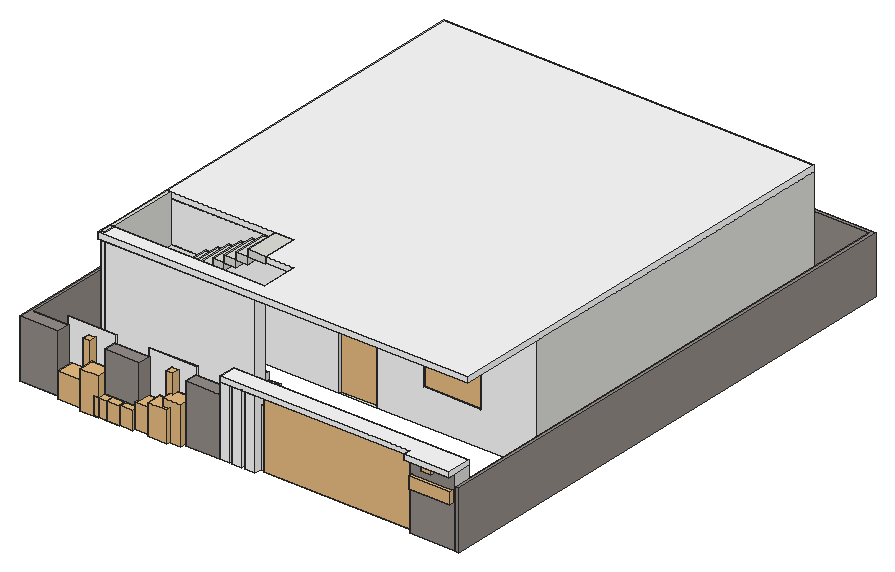
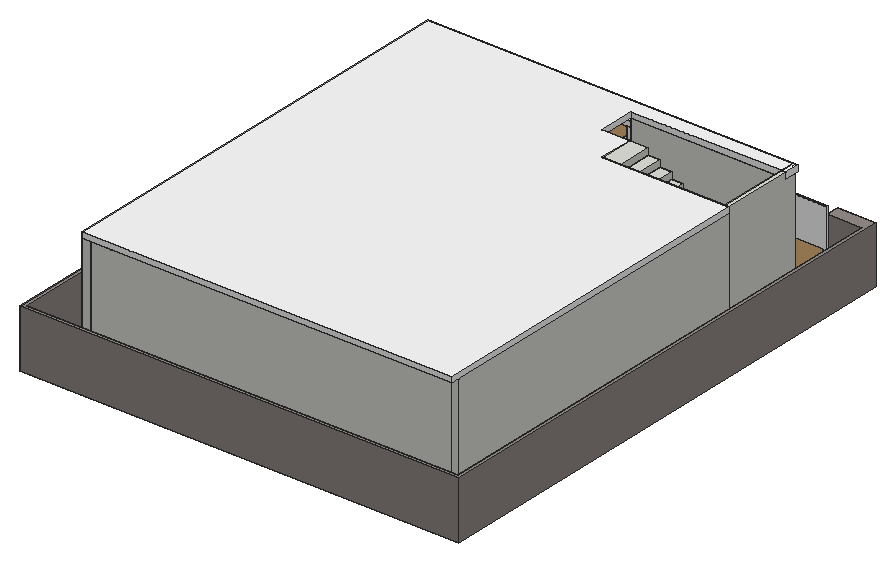
# SketchUp Ruby script. Lengths in inches.
U = 1.inch
M = Sketchup.active_model
def pt(a) = Geom::Point3d.new(a.map { |v| v * U })
def face(e, loops, mat)
  f = e.add_face(loops[0].map { |a| pt(a) })
  loops[1..].each { |l| e.add_face(l.map { |a| pt(a) }).erase! }
  f.material = f.back_material = mat if mat
  f
end
# faces: each face lists its corners as indices into pts; further lists are holes
def faces(e, pts, list, mat = nil) = list.each { |f| face(e, (f[0].is_a?(Array) ? f : [f]).map { |l| l.map { |i| pts[i] } }, mat) }
# xy, xz, yz: faces in a plane at the given z, y or x. An outline is a flat list of corners, or four numbers for a rectangle; further outlines are holes
def ring(l) = l.size == 4 ? [[l[0], l[1]], [l[2], l[1]], [l[2], l[3]], [l[0], l[3]]] : l.each_slice(2).to_a
def flat(e, list, mat, &to3) = list.each { |f| face(e, (f[0].is_a?(Array) ? f : [f]).map { |l| ring(l).map { |u, v| to3.(u, v) } }, mat) }
def xy(e, z, list, mat = nil) = flat(e, list, mat) { |x, y| [x, y, z] }
def xz(e, y, list, mat = nil) = flat(e, list, mat) { |x, z| [x, y, z] }
def yz(e, x, list, mat = nil) = flat(e, list, mat) { |y, z| [x, y, z] }
def lines(e, pts, list) = list.each { |a, b| e.add_line(pt(pts[a]), pt(pts[b])) }
# prism: a flat outline (further loops are holes) pulled along v
def prism(e, loops, v, mat = nil)
  f = face(e, loops, mat); d = Geom::Vector3d.new(v.map { |x| x * U })
  f.pushpull(f.normal.samedirection?(d) ? d.length : -d.length)
end
def box(e, o, s, mat = nil) = prism(e, [[o, [o[0] + s[0], o[1], o[2]], [o[0] + s[0], o[1] + s[1], o[2]], [o[0], o[1] + s[1], o[2]]]], [0, 0, s[2]], mat)
def at(x, y, z, deg = 0) = Geom::Transformation.translation(pt([x, y, z])) * Geom::Transformation.rotation(ORIGIN, Z_AXIS, deg.degrees)
def axes(o, x, y, z) = Geom::Transformation.new([*x, 0, *y, 0, *z, 0, *pt(o).to_a, 1])
def part(name) = M.definitions.add(name)
# library, detail: a bought-in or finely detailed component or shape, given as its bounding box
def library(name, o, s) = part(name).tap { |d| box(d.entities, o, s) }
def detail(e, o, s) = box(e.add_group.entities, o, s)
def put(e, d, t, mat = nil) = e.add_instance(d, t).tap { |i| i.material = mat if mat }
def group(e, t, mat = nil) = e.add_group.tap { |g| g.transformation = t; g.material = mat if mat }.entities
root = M.entities
M.materials.add("Ceramic Sand 8.13cm").color = [255, 255, 255]
M.materials.add("Foil Dark Green Matte 0.01cm").color = [255, 255, 255]
M.materials.add("Gold Gloss 0.02cm").color = [255, 255, 255]
M.materials.add("Leather Brown Alcantara 003 9.18cm").color = [255, 255, 255]
M.materials.add("Marble C 150cm").color = [150, 142, 138]
M.materials.add("Pp-1846-msg 17.72cm").color = [255, 255, 255]
c1 = library("Potted Plant 13",[-10,-7.28,0],[18.93,15.17,39.22])
c2 = library("Window Crafter Sliding",[0,-0.55,0],[60,4.49,60])
c3 = library("Door 243 065",[-19.36,-2.49,0],[38.72,4.98,81.96])
c4 = library("Group\#33",[0,0,0],[196.875,8,75.64])
c5 = library("Echinacea purpurea 001",[-10.375,-10.74,-1.26],[21.3,22.97,28.47])
c6 = library("Large Boxwood Plant 66-28",[-21.37,-20.87,0.32],[41.28,41.36,41.23])
c7 = part("Stair tread")
box(c7.entities,[0,0,0],[12,36,7])
c8 = part("Stair tread \#1")
box(c8.entities,[0,0,0],[19.0625,36,7])
c9 = library("Dalea purpurea 002",[-14.56,-13.24,-0.2],[28.56,28.68,23.96])
c10 = library("Iris versicolor 005",[-23.76,-20.68,-0.61],[47.57,44.31,52.43])
c11 = library("Group\#44",[0,0,0],[10.21,10.4,38.37])
c12 = library("sanath\#1",[-0.05,0,0],[42.98,11.6875,4])
c13 = library("Spot Light\#1",[-5.1,-5.1,-11.05],[10.2,10.2,11.05])
xy(root,6,[[1042,326.76,1088.95,344.76]])
xy(root,78.0625,[[1042,326.76,1088.95,344.76]])
xz(root,326.76,[[1042,6,1088.95,78.0625]],"Marble C 150cm")
xz(root,344.76,[[1042,6,1088.95,78.0625]])
yz(root,1042,[[326.76,6,344.76,78.0625]],"Marble C 150cm")
yz(root,1088.95,[[326.76,6,344.76,78.0625]])
put(root,c1,at(715.57,326.73,5.3))
g1 = group(root,at(672.95,472.76,6))
put(g1,c2,at(266.5625,2.73,36))
put(g1,c3,axes([198.48,4.93,0],[1,0,0],[0,1,0],[0,0,1.17128]))
g2 = group(g1,at(0,0,0))
xy(g2,0,[[179.1875,0,218.1875,9],[9,9,102,129],[106.5,9,226.5,129],[231,9,375,129],[9,133.5,102,262.5],
  [106.5,133.5,226.5,262.5],[231,133.5,375,262.5],[9,267,102,351],[106.5,267,226.5,351],[231,267,375,351]])
xy(g2,36,[[266.5625,0,326.5625,9]])
xy(g2,96,[[179.1875,0,218.1875,9],[266.5625,0,326.5625,9]])
xy(g2,120,[[[0,0,384,0,384,360,375,360,375,267,231,267,231,351,375,351,375,360,0,360,0,351,226.5,351,226.5,267,106.5,267,106.5,351,102,351,102,267,9,267,9,262.5,102,262.5,102,133.5,9,133.5,9,351,0,351],[106.5,9,106.5,129,226.5,129,226.5,9,231,9,231,129,375,129,375,9],[231,133.5,375,262.5],[106.5,133.5,226.5,262.5],[9,9,102,129]]])
xz(g2,0,[[[0,0,179.1875,0,179.1875,96,218.1875,96,218.1875,0,384,0,384,120,0,120],[266.5625,36,326.5625,96]]],"Pp-1846-msg 17.72cm")
xz(g2,9,[[9,0,102,120],[106.5,0,106.5,120,226.5,120,226.5,0,218.1875,0,218.1875,96,179.1875,96,179.1875,0],[226.5,0,231,120],[[231,0,375,120],[266.5625,36,326.5625,96]]])
xz(g2,129,[[9,0,102,120],[106.5,0,226.5,120],[231,0,375,120]])
xz(g2,133.5,[[9,0,102,120],[106.5,0,226.5,120],[231,0,375,120]])
xz(g2,262.5,[[9,0,102,120],[106.5,0,226.5,120],[231,0,375,120]])
xz(g2,267,[[9,0,102,120],[106.5,0,226.5,120],[231,0,375,120]])
xz(g2,351,[[0,0,9,120],[9,0,102,120],[102,0,106.5,120],[106.5,0,226.5,120],[231,0,375,120]])
xz(g2,360,[[0,0,375,120],[375,0,384,120]])
yz(g2,0,[[0,0,351,120],[351,0,360,120]])
yz(g2,9,[[9,0,129,120],[133.5,0,262.5,120],[262.5,0,267,120],[267,0,351,120]])
yz(g2,102,[[9,0,129,120],[133.5,0,262.5,120],[267,0,351,120]])
yz(g2,106.5,[[9,0,129,120],[133.5,0,262.5,120],[267,0,351,120]])
yz(g2,179.1875,[[0,0,9,96]])
yz(g2,218.1875,[[0,0,9,96]])
yz(g2,226.5,[[9,0,129,120],[133.5,0,262.5,120],[267,0,351,120]])
yz(g2,231,[[9,0,129,120],[133.5,0,262.5,120],[267,0,351,120]])
yz(g2,266.5625,[[0,36,9,96]])
yz(g2,326.5625,[[0,36,9,96]])
yz(g2,375,[[9,0,129,120],[133.5,0,262.5,120],[267,0,351,120],[351,0,360,120]])
yz(g2,384,[[0,0,360,120]])
put(root,c1,at(798.57,330.06,6))
put(root,c4,axes([885.36,332.88,6],[0.79562,0,0],[0,0.62,0],[0,0,0.95273]))
put(root,c5,axes([768.97,330.125,7.11],[0.82,0,0],[0,0.72,0],[0,0,0.88]))
put(root,c6,axes([740.5,323.13,5.85],[0.3294,0,0],[0,0.1769,0],[0,0,0.45091]))
put(root,c6,axes([753.31,323.13,5.85],[0.3294,0,0],[0,0.1769,0],[0,0,0.44878]))
put(root,c6,axes([727.06,323.13,5.85],[0.3294,0,0],[0,0.1769,0],[0,0,0.44797]))
g3 = group(root,at(672.95,398.76,6))
xy(g3,0,[[0,-12,4.5,74]])
xy(g3,126,[[0,-12,4.5,74]])
xz(g3,-12,[[0,0,4.5,126]],"Pp-1846-msg 17.72cm")
xz(g3,74,[[0,0,4.5,126]])
yz(g3,0,[[-12,0,74,126]])
yz(g3,4.5,[[-12,0,74,126]])
g4 = group(root,at(677.45,398.76,6))
box(g4,[0,0,70],[36,74,7])
put(g4,c7,at(36,38,77))
put(g4,c7,at(132,0,7))
put(g4,c7,at(108,0,21))
put(g4,c7,at(120,0,14))
put(g4,c7,at(144,0,0))
put(g4,c7,at(60,38,91))
put(g4,c7,at(84,38,105))
put(g4,c7,at(96,38,112))
put(g4,c7,at(48,38,84))
put(g4,c8,at(108,38,119))
put(g4,c7,at(72,38,98))
put(g4,c7,at(48,0,56))
put(g4,c7,at(60,0,49))
put(g4,c7,at(36,0,63))
put(g4,c7,at(84,0,35))
put(g4,c7,at(96,0,28))
put(g4,c7,at(72,0,42))
g5 = group(root,at(677.45,386.76,6))
xy(g5,0,[[0,0,156,12]])
xy(g5,120,[[0,0,156,12]])
xz(g5,0,[[0,0,156,120]],"Pp-1846-msg 17.72cm")
xz(g5,12,[[0,0,156,120]])
yz(g5,0,[[0,0,12,120]])
yz(g5,156,[[0,0,12,120]],"Pp-1846-msg 17.72cm")
g6 = group(root,at(636.95,326.76,6),"Marble C 150cm")
prism(g6,[[[0,0,0],[0,542,0],[456,542,0],[456,0,0],[452,0,0],[452,538,0],[4,538,0],[4,13.375,0],[40,13.375,0],[40,0,0]]],[0,0,60],"Marble C 150cm")
g7 = group(root,at(724.95,326.76,6),"Marble C 150cm")
box(g7,[0,0,0],[36,13.375,60],"Marble C 150cm")
g8 = group(root,at(808.95,326.76,6))
box(g8,[0,0,0],[36,13.375,60],"Marble C 150cm")
g9 = group(root,at(675.95,340.13,6),"Leather Brown Alcantara 003 9.18cm")
box(g9,[0,0,0],[50,1.25,67.625])
g10 = group(root,at(759.95,340.13,6),"Leather Brown Alcantara 003 9.18cm")
box(g10,[0,0,0],[50,1.25,67.625])
g11 = group(root,at(844.95,334.01,6))
box(g11,[0,0,0],[40.42,10.75,60])
g12 = group(root,at(844.95,326.76,6),"Ceramic Sand 8.13cm")
prism(g12,[[[10.21,0,0],[10.21,7.25,0],[10.21,7.25,59.8125],[10.21,18,59.8125],[10.21,18,72.0625],[10.21,0,72.0625]]],[-10.21,0,0])
g13 = group(root,at(857.7,326.76,6),"Ceramic Sand 8.13cm")
prism(g13,[[[10.21,0,0],[10.21,7.25,0],[10.21,7.25,59.8125],[10.21,18,59.8125],[10.21,18,72.0625],[10.21,0,72.0625]]],[-10.21,0,0])
g14 = group(root,at(871.26,326.76,6),"Ceramic Sand 8.13cm")
prism(g14,[[[10.21,0,0],[10.21,7.25,0],[10.21,7.25,59.8125],[10.21,18,59.8125],[10.21,18,72.0625],[10.21,0,72.0625]]],[-10.21,0,0])
put(root,c9,axes([785.87,326.87,6.26],[0.71,0,0],[0,0.54,0],[0,0,1.31]))
put(root,c10,axes([698.85,331,6.31],[0.7686,0,0],[0,0.43963,0],[0,0,0.5032]))
put(root,c11,axes([697.99,332.65,36.89],[0.72,0,0],[0,0.72,0],[0,0,0.72]))
put(root,c11,axes([784.12,332.65,36.89],[0.72,0,0],[0,0.72,0],[0,0,0.72]))
put(root,c12,axes([1044.17,326.76,50.36],[1,0,0],[0,0,1],[0,-1,0]),"Gold Gloss 0.02cm")
put(root,c13,axes([1065.47,323.95,78.05],[1,0,0],[0,1,0],[0,0,0.37]))
g15 = group(root,at(844.95,326.76,78.0625),"Ceramic Sand 8.13cm")
prism(g15,[[[197.05,0,0],[0,0,0],[0,18,0],[244,18,0],[244,-7.875,0],[197.05,-7.875,0]]],[0,0,5.0625])
g16 = group(root,at(672.95,472.76,126),"Foil Dark Green Matte 0.01cm")
prism(g16,[[[384,-89.125,0],[0,-89.125,0],[0,-74,0],[160.5,-74,0],[160.5,-36,0],[131.5625,-36,0],[131.5625,0,0],[4.5,0,0],[0,0,0],[0,360,0],[384,360,0]]],[0,0,6])
